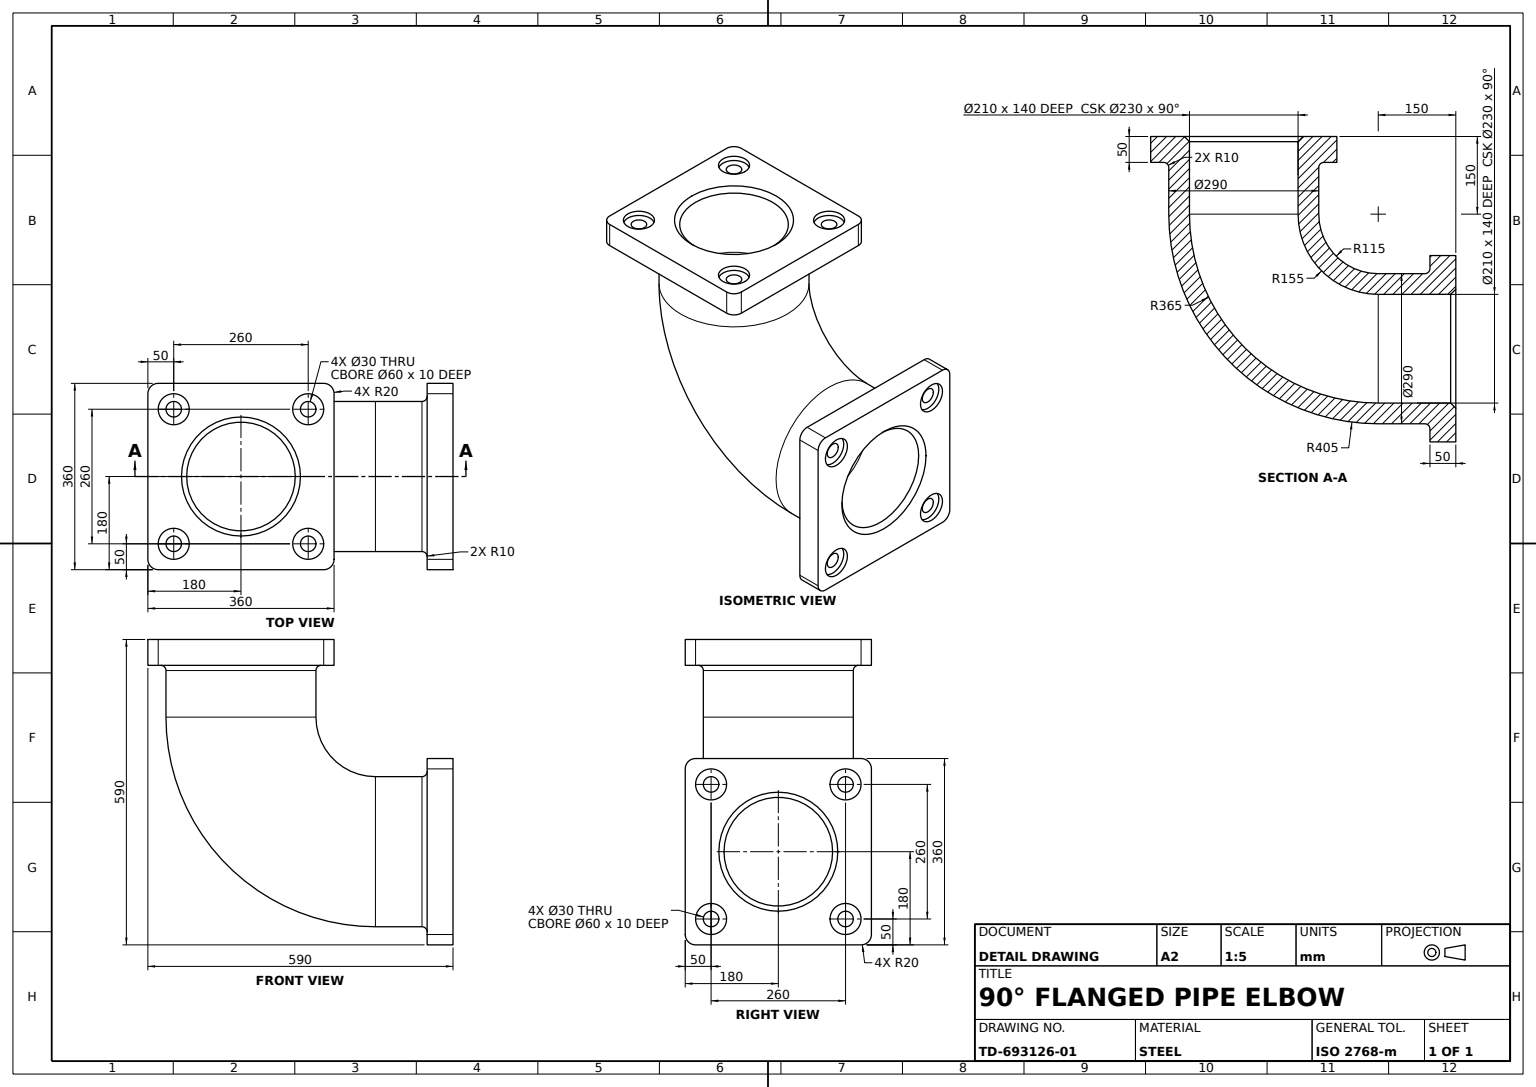
solid
v1 (0,260,215)
v2 (0,260,505)
e1 v1 v2 CIRCLE(AX(P(0,260,360),D(0,1,0),D(0,0,1)),145)
v3 (0,145,100)
e2 v3 v1 CIRCLE(AX(P(0,260,100),D(-1,0,0),D(0,0,1)),115)
v4 (0,-145,100)
e3 v3 v4 CIRCLE(AX(P(0,0,100),D(0,0,1),D(0,-1,0)),145)
e4 v4 v2 CIRCLE(AX(P(0,260,100),D(-1,0,0),D(0,0,1)),405)
face TORUS(AX(P(0,260,100),D(-1,0,0),D(0,0,1)),260,145) [-e1 -e2 e3 e4]
v5 (-100,130,-40)
v6 (-160,130,-40)
e5 v5 v6 CIRCLE(AX(P(-130,130,-40),D(0,0,-1),D(-1,0,0)),30)
v7 (-100,130,-50)
e6 v5 v7 LINE
v8 (-160,130,-50)
e7 v7 v8 CIRCLE(AX(P(-130,130,-50),D(0,0,-1),D(-1,0,0)),30)
e8 v6 v8 LINE
face CYL(AX(P(-130,130,-40),D(0,0,-1),D(-1,0,0)),30) rev [-e5 e6 e7 -e8]
e9 v6 v5 CIRCLE(AX(P(-130,130,-40),D(0,0,-1),D(-1,0,0)),30)
e10 v8 v7 CIRCLE(AX(P(-130,130,-50),D(0,0,-1),D(-1,0,0)),30)
face CYL(AX(P(-130,130,-40),D(0,0,-1),D(-1,0,0)),30) rev [-e9 e8 e10 -e6]
v9 (-130,400,200)
v10 (-130,410,200)
e11 v9 v10 LINE
v11 (-130,400,260)
e12 v11 v9 CIRCLE(AX(P(-130,400,230),D(0,1,0),D(0,0,1)),30)
v12 (-130,410,260)
e13 v11 v12 LINE
e14 v12 v10 CIRCLE(AX(P(-130,410,230),D(0,1,0),D(0,0,1)),30)
face CYL(AX(P(-130,400,230),D(0,1,0),D(0,0,1)),30) rev [-e11 -e12 e13 e14]
v13 (-130,400,520)
v14 (-130,400,460)
e15 v13 v14 CIRCLE(AX(P(-130,400,490),D(0,1,0),D(0,0,1)),30)
v15 (-130,410,520)
e16 v13 v15 LINE
v16 (-130,410,460)
e17 v15 v16 CIRCLE(AX(P(-130,410,490),D(0,1,0),D(0,0,1)),30)
e18 v14 v16 LINE
face CYL(AX(P(-130,400,490),D(0,1,0),D(0,0,1)),30) rev [-e15 e16 e17 -e18]
e19 v14 v13 CIRCLE(AX(P(-130,400,490),D(0,1,0),D(0,0,1)),30)
v17 (-130,400,505)
v18 (-130,400,475)
e20 v17 v18 CIRCLE(AX(P(-130,400,490),D(0,1,0),D(0,0,1)),15)
e21 v18 v17 CIRCLE(AX(P(-130,400,490),D(0,1,0),D(0,0,1)),15)
face PLANE(AX(P(-130,400,490),D(0,1,0),D(0,0,1))) [e19 e15] [-e20 -e21]
v19 (-180,-160,-50)
v20 (-180,-160,0)
e22 v19 v20 LINE
v21 (-180,160,0)
e23 v21 v20 LINE
v22 (-180,160,-50)
e24 v21 v22 LINE
e25 v22 v19 LINE
face PLANE(AX(P(-180,180,-50),D(-1,0,0),D(0,-1,0))) [e22 -e23 e24 e25]
v23 (-130,360,475)
e26 v18 v23 LINE
v24 (-130,360,505)
e27 v24 v23 CIRCLE(AX(P(-130,360,490),D(0,1,0),D(0,0,1)),15)
e28 v17 v24 LINE
face CYL(AX(P(-130,410,490),D(0,-1,0),D(0,0,-1)),15) rev [e20 e26 -e27 -e28]
v25 (130,400,200)
v26 (130,410,200)
e29 v25 v26 LINE
v27 (130,400,260)
e30 v27 v25 CIRCLE(AX(P(130,400,230),D(0,1,0),D(0,0,1)),30)
v28 (130,410,260)
e31 v27 v28 LINE
e32 v28 v26 CIRCLE(AX(P(130,410,230),D(0,1,0),D(0,0,1)),30)
face CYL(AX(P(130,400,230),D(0,1,0),D(0,0,1)),30) rev [-e29 -e30 e31 e32]
v29 (0,350,215)
e33 v1 v29 LINE
v30 (0,350,505)
e34 v2 v30 LINE
e35 v30 v29 CIRCLE(AX(P(0,350,360),D(0,-1,0),D(0,0,1)),145)
face CYL(AX(P(0,260,360),D(0,1,0),D(0,0,1)),145) [-e33 e1 e34 e35]
v31 (-115,-130,-40)
v32 (-145,-130,-40)
e36 v31 v32 CIRCLE(AX(P(-130,-130,-40),D(0,0,1),D(-1,0,0)),15)
v33 (-115,-130,0)
e37 v31 v33 LINE
v34 (-145,-130,0)
e38 v33 v34 CIRCLE(AX(P(-130,-130,0),D(0,0,1),D(1,0,0)),15)
e39 v32 v34 LINE
face CYL(AX(P(-130,-130,-50),D(0,0,1),D(1,0,0)),15) rev [-e36 e37 e38 -e39]
v35 (115,0,-50)
v36 (-115,0,-50)
e40 v35 v36 CIRCLE(AX(P(0,0,-50),D(0,0,1),D(1,0,0)),115)
v37 (105,0,-40)
e41 v37 v35 LINE
v38 (-105,0,-40)
e42 v38 v37 CIRCLE(AX(P(0,0,-40),D(0,0,-1),D(1,0,0)),105)
e43 v38 v36 LINE
face CONE(AX(P(0,0,-50),D(0,0,-1),D(-1,0,0)),115,0.785398163) rev [-e40 -e41 -e42 e43]
v39 (160,130,-40)
v40 (100,130,-40)
e44 v39 v40 CIRCLE(AX(P(130,130,-40),D(0,0,-1),D(-1,0,0)),30)
v41 (160,130,-50)
e45 v39 v41 LINE
v42 (100,130,-50)
e46 v41 v42 CIRCLE(AX(P(130,130,-50),D(0,0,-1),D(-1,0,0)),30)
e47 v40 v42 LINE
face CYL(AX(P(130,130,-40),D(0,0,-1),D(-1,0,0)),30) rev [-e44 e45 e46 -e47]
v43 (180,410,520)
v44 (180,410,200)
e48 v43 v44 LINE
v45 (160,410,180)
e49 v44 v45 CIRCLE(AX(P(160,410,200),D(0,1,0),D(0,0,1)),20)
v46 (-160,410,180)
e50 v45 v46 LINE
v47 (-180,410,200)
e51 v46 v47 CIRCLE(AX(P(-160,410,200),D(0,1,0),D(0,0,1)),20)
v48 (-180,410,520)
e52 v47 v48 LINE
v49 (-160,410,540)
e53 v48 v49 CIRCLE(AX(P(-160,410,520),D(0,1,0),D(0,0,1)),20)
v50 (160,410,540)
e54 v49 v50 LINE
e55 v50 v43 CIRCLE(AX(P(160,410,520),D(0,1,0),D(0,0,1)),20)
e56 v10 v12 CIRCLE(AX(P(-130,410,230),D(0,1,0),D(0,0,1)),30)
v51 (130,410,520)
v52 (130,410,460)
e57 v51 v52 CIRCLE(AX(P(130,410,490),D(0,1,0),D(0,0,1)),30)
e58 v52 v51 CIRCLE(AX(P(130,410,490),D(0,1,0),D(0,0,1)),30)
e59 v26 v28 CIRCLE(AX(P(130,410,230),D(0,1,0),D(0,0,1)),30)
v53 (0,410,245)
v54 (0,410,475)
e60 v53 v54 CIRCLE(AX(P(0,410,360),D(0,-1,0),D(0,0,1)),115)
e61 v54 v53 CIRCLE(AX(P(0,410,360),D(0,-1,0),D(0,0,1)),115)
e62 v16 v15 CIRCLE(AX(P(-130,410,490),D(0,1,0),D(0,0,1)),30)
face PLANE(AX(P(0,410,0),D(0,1,0),D(0,0,1))) [e48 e49 e50 e51 e52 e53 e54 e55] [-e56 -e14] [-e57 -e58] [-e59 -e32] [e60 e61] [-e17 -e62]
v55 (105,0,100)
e63 v37 v55 LINE
v56 (0,105,100)
e64 v56 v55 CIRCLE(AX(P(0,0,100),D(0,0,-1),D(0,-1,0)),105)
v57 (-105,0,100)
e65 v57 v56 CIRCLE(AX(P(0,0,100),D(0,0,-1),D(0,-1,0)),105)
e66 v38 v57 LINE
face CYL(AX(P(0,0,-50),D(0,0,1),D(1,0,0)),105) rev [e42 e63 -e64 -e65 -e66]
v58 (0,-105,100)
v59 (0,260,465)
e67 v58 v59 CIRCLE(AX(P(0,260,100),D(-1,0,0),D(0,0,1)),365)
v60 (0,260,255)
e68 v60 v59 CIRCLE(AX(P(0,260,360),D(0,-1,0),D(0,0,1)),105)
e69 v56 v60 CIRCLE(AX(P(0,260,100),D(-1,0,0),D(0,0,1)),155)
e70 v55 v58 CIRCLE(AX(P(0,0,100),D(0,0,-1),D(0,-1,0)),105)
face TORUS(AX(P(0,260,100),D(-1,0,0),D(0,0,1)),260,105) rev [e67 -e68 -e69 e64 e70]
e71 v37 v38 CIRCLE(AX(P(0,0,-40),D(0,0,-1),D(1,0,0)),105)
e72 v36 v35 CIRCLE(AX(P(0,0,-50),D(0,0,1),D(1,0,0)),115)
face CONE(AX(P(0,0,-50),D(0,0,-1),D(-1,0,0)),115,0.785398163) rev [-e71 e41 -e72 -e43]
v61 (0,360,205)
v62 (0,360,515)
e73 v61 v62 CIRCLE(AX(P(0,360,360),D(0,1,0),D(0,0,1)),155)
e74 v61 v29 CIRCLE(AX(P(0,350,205),D(1,0,0),D(0,0,-1)),10)
e75 v62 v30 CIRCLE(AX(P(0,350,515),D(-1,0,0),D(0,0,1)),10)
face TORUS(AX(P(0,350,360),D(0,1,0),D(0,0,1)),155,10) rev [-e73 e74 -e35 -e75]
v63 (160,180,0)
v64 (160,180,-50)
e76 v63 v64 LINE
v65 (-160,180,-50)
e77 v64 v65 LINE
v66 (-160,180,0)
e78 v65 v66 LINE
e79 v63 v66 LINE
face PLANE(AX(P(-180,180,-50),D(0,1,0),D(0,0,1))) [e76 e77 e78 -e79]
v67 (-160,-180,0)
v68 (-160,-180,-50)
e80 v67 v68 LINE
v69 (160,-180,-50)
e81 v68 v69 LINE
v70 (160,-180,0)
e82 v69 v70 LINE
e83 v67 v70 LINE
face PLANE(AX(P(-180,-180,-50),D(0,-1,0),D(0,0,-1))) [e80 e81 e82 -e83]
e84 v59 v60 CIRCLE(AX(P(0,260,360),D(0,-1,0),D(0,0,1)),105)
e85 v58 v57 CIRCLE(AX(P(0,0,100),D(0,0,-1),D(0,-1,0)),105)
face TORUS(AX(P(0,260,100),D(-1,0,0),D(0,0,1)),260,105) rev [e65 e69 -e84 -e67 e85]
v71 (0,-145,10)
v72 (145,0,10)
e86 v71 v72 CIRCLE(AX(P(0,0,10),D(0,0,1),D(1,0,0)),145)
v73 (0,145,10)
e87 v72 v73 CIRCLE(AX(P(0,0,10),D(0,0,1),D(1,0,0)),145)
e88 v73 v3 LINE
e89 v4 v3 CIRCLE(AX(P(0,0,100),D(0,0,1),D(0,-1,0)),145)
e90 v71 v4 LINE
face CYL(AX(P(0,0,0),D(0,0,1),D(0,-1,0)),145) [e86 e87 e88 -e89 -e90]
v74 (-160,360,540)
v75 (-180,360,520)
e91 v74 v75 CIRCLE(AX(P(-160,360,520),D(0,-1,0),D(0,0,1)),20)
e92 v49 v74 LINE
e93 v75 v48 LINE
face CYL(AX(P(-160,410,520),D(0,-1,0),D(0,0,-1)),20) [-e91 -e92 -e53 -e93]
v76 (145,130,0)
v77 (115,130,0)
e94 v76 v77 CIRCLE(AX(P(130,130,0),D(0,0,1),D(1,0,0)),15)
v78 (115,130,-40)
e95 v78 v77 LINE
v79 (145,130,-40)
e96 v79 v78 CIRCLE(AX(P(130,130,-40),D(0,0,1),D(-1,0,0)),15)
e97 v79 v76 LINE
face CYL(AX(P(130,130,-50),D(0,0,1),D(1,0,0)),15) rev [e94 -e95 -e96 e97]
e98 v23 v24 CIRCLE(AX(P(-130,360,490),D(0,1,0),D(0,0,1)),15)
face CYL(AX(P(-130,410,490),D(0,-1,0),D(0,0,-1)),15) rev [e21 e28 -e98 -e26]
v80 (100,-130,-40)
v81 (160,-130,-40)
e99 v80 v81 CIRCLE(AX(P(130,-130,-40),D(0,0,-1),D(-1,0,0)),30)
e100 v81 v80 CIRCLE(AX(P(130,-130,-40),D(0,0,-1),D(-1,0,0)),30)
v82 (115,-130,-40)
v83 (145,-130,-40)
e101 v82 v83 CIRCLE(AX(P(130,-130,-40),D(0,0,1),D(-1,0,0)),15)
e102 v83 v82 CIRCLE(AX(P(130,-130,-40),D(0,0,1),D(-1,0,0)),15)
face PLANE(AX(P(130,-130,-40),D(0,0,-1),D(-1,0,0))) [e99 e100] [e101 e102]
v84 (160,360,540)
e103 v84 v50 LINE
v85 (180,360,520)
e104 v85 v84 CIRCLE(AX(P(160,360,520),D(0,-1,0),D(0,0,1)),20)
e105 v43 v85 LINE
face CYL(AX(P(160,410,520),D(0,-1,0),D(0,0,-1)),20) [-e103 -e104 -e105 -e55]
e106 v42 v41 CIRCLE(AX(P(130,130,-50),D(0,0,-1),D(-1,0,0)),30)
e107 v68 v19 CIRCLE(AX(P(-160,-160,-50),D(0,0,-1),D(1,0,0)),20)
e108 v22 v65 CIRCLE(AX(P(-160,160,-50),D(0,0,-1),D(1,0,0)),20)
v86 (180,160,-50)
e109 v64 v86 CIRCLE(AX(P(160,160,-50),D(0,0,-1),D(1,0,0)),20)
v87 (180,-160,-50)
e110 v87 v86 LINE
e111 v87 v69 CIRCLE(AX(P(160,-160,-50),D(0,0,-1),D(1,0,0)),20)
v88 (160,-130,-50)
v89 (100,-130,-50)
e112 v88 v89 CIRCLE(AX(P(130,-130,-50),D(0,0,-1),D(-1,0,0)),30)
e113 v89 v88 CIRCLE(AX(P(130,-130,-50),D(0,0,-1),D(-1,0,0)),30)
v90 (-160,-130,-50)
v91 (-100,-130,-50)
e114 v90 v91 CIRCLE(AX(P(-130,-130,-50),D(0,0,-1),D(-1,0,0)),30)
e115 v91 v90 CIRCLE(AX(P(-130,-130,-50),D(0,0,-1),D(-1,0,0)),30)
face PLANE(AX(P(0,0,-50),D(0,0,1),D(1,0,0))) rev [-e106 -e46] [e40 e72] [e107 -e25 e108 -e77 e109 -e110 e111 -e81] [-e7 -e10] [-e112 -e113] [-e114 -e115]
v92 (0,400,255)
e116 v92 v53 LINE
v93 (0,400,465)
e117 v93 v54 LINE
e118 v92 v93 CIRCLE(AX(P(0,400,360),D(0,1,0),D(0,0,1)),105)
face CONE(AX(P(0,400,360),D(0,1,0),D(0,0,1)),105,0.785398163) rev [e116 -e61 -e117 -e118]
v94 (-160,-130,-40)
v95 (-100,-130,-40)
e119 v94 v95 CIRCLE(AX(P(-130,-130,-40),D(0,0,-1),D(-1,0,0)),30)
e120 v94 v90 LINE
e121 v95 v91 LINE
face CYL(AX(P(-130,-130,-40),D(0,0,-1),D(-1,0,0)),30) rev [-e119 e120 e114 -e121]
e122 v40 v39 CIRCLE(AX(P(130,130,-40),D(0,0,-1),D(-1,0,0)),30)
face CYL(AX(P(130,130,-40),D(0,0,-1),D(-1,0,0)),30) rev [-e45 -e122 e47 e106]
e123 v32 v31 CIRCLE(AX(P(-130,-130,-40),D(0,0,1),D(-1,0,0)),15)
e124 v95 v94 CIRCLE(AX(P(-130,-130,-40),D(0,0,-1),D(-1,0,0)),30)
face PLANE(AX(P(-130,-130,-40),D(0,0,-1),D(-1,0,0))) [e36 e123] [e119 e124]
e125 v29 v30 CIRCLE(AX(P(0,350,360),D(0,-1,0),D(0,0,1)),145)
e126 v2 v1 CIRCLE(AX(P(0,260,360),D(0,1,0),D(0,0,1)),145)
face CYL(AX(P(0,260,360),D(0,1,0),D(0,0,1)),145) [e125 -e34 e126 e33]
e127 v20 v67 CIRCLE(AX(P(-160,-160,0),D(0,0,1),D(1,0,0)),20)
face CYL(AX(P(-160,-160,-50),D(0,0,1),D(1,0,0)),20) [-e107 -e80 -e127 -e22]
v96 (180,160,0)
e128 v86 v96 LINE
v97 (180,-160,0)
e129 v97 v96 LINE
e130 v97 v87 LINE
face PLANE(AX(P(180,180,-50),D(1,0,0),D(0,1,0))) [e110 e128 -e129 e130]
face TORUS(AX(P(0,260,100),D(-1,0,0),D(0,0,1)),260,145) [-e126 -e4 e89 e2]
e131 v81 v88 LINE
e132 v80 v89 LINE
face CYL(AX(P(130,-130,-40),D(0,0,-1),D(-1,0,0)),30) rev [-e100 e131 e112 -e132]
v98 (130,400,215)
v99 (130,360,215)
e133 v98 v99 LINE
v100 (130,360,245)
e134 v100 v99 CIRCLE(AX(P(130,360,230),D(0,1,0),D(0,0,1)),15)
v101 (130,400,245)
e135 v101 v100 LINE
e136 v101 v98 CIRCLE(AX(P(130,400,230),D(0,1,0),D(0,0,1)),15)
face CYL(AX(P(130,410,230),D(0,-1,0),D(0,0,-1)),15) rev [e133 -e134 -e135 e136]
face CYL(AX(P(-130,-130,-40),D(0,0,-1),D(-1,0,0)),30) rev [e121 e115 -e120 -e124]
face CYL(AX(P(0,0,-50),D(0,0,1),D(1,0,0)),105) rev [-e85 -e70 -e63 e71 e66]
e137 v66 v21 CIRCLE(AX(P(-160,160,0),D(0,0,1),D(1,0,0)),20)
face CYL(AX(P(-160,160,-50),D(0,0,1),D(1,0,0)),20) [-e78 -e108 -e24 -e137]
e138 v59 v93 LINE
e139 v60 v92 LINE
face CYL(AX(P(0,260,360),D(0,1,0),D(0,0,1)),105) rev [e118 -e138 e84 e139]
v102 (160,360,180)
e140 v45 v102 LINE
v103 (-160,360,180)
e141 v102 v103 LINE
e142 v103 v46 LINE
face PLANE(AX(P(-180,410,180),D(0,0,1),D(1,0,0))) rev [e140 e141 e142 -e50]
e143 v34 v33 CIRCLE(AX(P(-130,-130,0),D(0,0,1),D(1,0,0)),15)
face CYL(AX(P(-130,-130,-50),D(0,0,1),D(1,0,0)),15) rev [e143 -e37 -e123 e39]
v104 (130,400,475)
v105 (130,360,475)
e144 v104 v105 LINE
v106 (130,360,505)
e145 v106 v105 CIRCLE(AX(P(130,360,490),D(0,1,0),D(0,0,1)),15)
v107 (130,400,505)
e146 v107 v106 LINE
e147 v107 v104 CIRCLE(AX(P(130,400,490),D(0,1,0),D(0,0,1)),15)
face CYL(AX(P(130,410,490),D(0,-1,0),D(0,0,-1)),15) rev [e144 -e145 -e146 e147]
v108 (-130,400,215)
v109 (-130,400,245)
e148 v108 v109 CIRCLE(AX(P(-130,400,230),D(0,1,0),D(0,0,1)),15)
v110 (-130,360,245)
e149 v109 v110 LINE
v111 (-130,360,215)
e150 v111 v110 CIRCLE(AX(P(-130,360,230),D(0,1,0),D(0,0,1)),15)
e151 v108 v111 LINE
face CYL(AX(P(-130,410,230),D(0,-1,0),D(0,0,-1)),15) rev [e148 e149 -e150 -e151]
e152 v62 v61 CIRCLE(AX(P(0,360,360),D(0,1,0),D(0,0,1)),155)
face TORUS(AX(P(0,350,360),D(0,1,0),D(0,0,1)),155,10) rev [-e74 -e152 e75 -e125]
e153 v9 v11 CIRCLE(AX(P(-130,400,230),D(0,1,0),D(0,0,1)),30)
e154 v109 v108 CIRCLE(AX(P(-130,400,230),D(0,1,0),D(0,0,1)),15)
face PLANE(AX(P(-130,400,230),D(0,1,0),D(0,0,1))) [e12 e153] [-e148 -e154]
v112 (180,360,200)
e155 v112 v44 LINE
e156 v85 v112 LINE
face PLANE(AX(P(180,410,180),D(-1,0,0),D(0,0,1))) rev [e155 -e48 e105 e156]
e157 v99 v100 CIRCLE(AX(P(130,360,230),D(0,1,0),D(0,0,1)),15)
e158 v98 v101 CIRCLE(AX(P(130,400,230),D(0,1,0),D(0,0,1)),15)
face CYL(AX(P(130,410,230),D(0,-1,0),D(0,0,-1)),15) rev [e135 -e157 -e133 e158]
v113 (-115,130,-40)
v114 (-145,130,-40)
e159 v113 v114 CIRCLE(AX(P(-130,130,-40),D(0,0,1),D(-1,0,0)),15)
v115 (-115,130,0)
e160 v113 v115 LINE
v116 (-145,130,0)
e161 v115 v116 CIRCLE(AX(P(-130,130,0),D(0,0,1),D(1,0,0)),15)
e162 v114 v116 LINE
face CYL(AX(P(-130,130,-50),D(0,0,1),D(1,0,0)),15) rev [-e159 e160 e161 -e162]
v117 (-180,360,200)
e163 v117 v103 CIRCLE(AX(P(-160,360,200),D(0,-1,0),D(0,0,1)),20)
e164 v47 v117 LINE
face CYL(AX(P(-160,410,200),D(0,-1,0),D(0,0,-1)),20) [-e163 -e164 -e51 -e142]
e165 v70 v97 CIRCLE(AX(P(160,-160,0),D(0,0,1),D(1,0,0)),20)
face CYL(AX(P(160,-160,-50),D(0,0,1),D(1,0,0)),20) [-e82 -e111 -e130 -e165]
face CYL(AX(P(130,-130,-40),D(0,0,-1),D(-1,0,0)),30) rev [e113 -e131 -e99 e132]
e166 v116 v115 CIRCLE(AX(P(-130,130,0),D(0,0,1),D(1,0,0)),15)
e167 v114 v113 CIRCLE(AX(P(-130,130,-40),D(0,0,1),D(-1,0,0)),15)
face CYL(AX(P(-130,130,-50),D(0,0,1),D(1,0,0)),15) rev [e166 -e160 -e167 e162]
e168 v105 v106 CIRCLE(AX(P(130,360,490),D(0,1,0),D(0,0,1)),15)
e169 v117 v75 LINE
e170 v102 v112 CIRCLE(AX(P(160,360,200),D(0,-1,0),D(0,0,1)),20)
e171 v74 v84 LINE
e172 v110 v111 CIRCLE(AX(P(-130,360,230),D(0,1,0),D(0,0,1)),15)
face PLANE(AX(P(0,360,0),D(0,1,0),D(0,0,1))) rev [e152 e73] [e168 e145] [e91 -e169 e163 -e141 e170 -e156 e104 -e171] [e172 e150] [e134 e157] [e98 e27]
face CYL(AX(P(-130,400,230),D(0,1,0),D(0,0,1)),30) rev [-e153 e11 e56 -e13]
face PLANE(AX(P(-180,410,540),D(0,0,-1),D(-1,0,0))) rev [e92 e171 e103 -e54]
e173 v96 v63 CIRCLE(AX(P(160,160,0),D(0,0,1),D(1,0,0)),20)
v118 (155,0,0)
v119 (-155,0,0)
e174 v118 v119 CIRCLE(AX(P(0,0,0),D(0,0,-1),D(1,0,0)),155)
e175 v119 v118 CIRCLE(AX(P(0,0,0),D(0,0,-1),D(1,0,0)),155)
e176 v77 v76 CIRCLE(AX(P(130,130,0),D(0,0,1),D(1,0,0)),15)
v120 (115,-130,0)
v121 (145,-130,0)
e177 v120 v121 CIRCLE(AX(P(130,-130,0),D(0,0,1),D(1,0,0)),15)
e178 v121 v120 CIRCLE(AX(P(130,-130,0),D(0,0,1),D(1,0,0)),15)
face PLANE(AX(P(0,0,0),D(0,0,1),D(1,0,0))) [-e143 -e38] [-e161 -e166] [e165 e129 e173 e79 e137 e23 e127 e83] [e174 e175] [-e176 -e94] [-e177 -e178]
e179 v25 v27 CIRCLE(AX(P(130,400,230),D(0,1,0),D(0,0,1)),30)
face CYL(AX(P(130,400,230),D(0,1,0),D(0,0,1)),30) rev [-e31 -e179 e29 e59]
face CYL(AX(P(160,160,-50),D(0,0,1),D(1,0,0)),20) [-e173 -e128 -e109 -e76]
face CYL(AX(P(160,410,200),D(0,-1,0),D(0,0,-1)),20) [-e155 -e170 -e140 -e49]
v122 (-145,0,10)
e180 v73 v122 CIRCLE(AX(P(0,0,10),D(0,0,1),D(1,0,0)),145)
e181 v122 v71 CIRCLE(AX(P(0,0,10),D(0,0,1),D(1,0,0)),145)
face CYL(AX(P(0,0,0),D(0,0,1),D(0,-1,0)),145) [-e88 e180 e181 e90 -e3]
e182 v93 v92 CIRCLE(AX(P(0,400,360),D(0,1,0),D(0,0,1)),105)
face CONE(AX(P(0,400,360),D(0,1,0),D(0,0,1)),105,0.785398163) rev [-e116 -e182 e117 -e60]
e183 v72 v118 CIRCLE(AX(P(155,0,10),D(0,-1,0),D(0,0,-1)),10)
e184 v122 v119 CIRCLE(AX(P(-155,0,10),D(0,1,0),D(-1,0,0)),10)
face TORUS(AX(P(0,0,10),D(0,0,1),D(1,0,0)),155,10) rev [-e180 -e87 e183 -e175 -e184]
face PLANE(AX(P(-130,130,-40),D(0,0,-1),D(-1,0,0))) [e9 e5] [e159 e167]
v123 (130,400,520)
v124 (130,400,460)
e185 v123 v124 CIRCLE(AX(P(130,400,490),D(0,1,0),D(0,0,1)),30)
e186 v124 v123 CIRCLE(AX(P(130,400,490),D(0,1,0),D(0,0,1)),30)
e187 v104 v107 CIRCLE(AX(P(130,400,490),D(0,1,0),D(0,0,1)),15)
face PLANE(AX(P(130,400,490),D(0,1,0),D(0,0,1))) [e185 e186] [-e147 -e187]
face CYL(AX(P(-130,410,230),D(0,-1,0),D(0,0,-1)),15) rev [-e172 -e149 e154 e151]
face PLANE(AX(P(130,400,230),D(0,1,0),D(0,0,1))) [e30 e179] [-e158 -e136]
e188 v78 v79 CIRCLE(AX(P(130,130,-40),D(0,0,1),D(-1,0,0)),15)
face PLANE(AX(P(130,130,-40),D(0,0,-1),D(-1,0,0))) [e96 e188] [e44 e122]
e189 v124 v52 LINE
e190 v123 v51 LINE
face CYL(AX(P(130,400,490),D(0,1,0),D(0,0,1)),30) rev [e189 e58 -e190 -e186]
face CYL(AX(P(-130,400,490),D(0,1,0),D(0,0,1)),30) rev [e18 e62 -e16 -e19]
face CYL(AX(P(130,400,490),D(0,1,0),D(0,0,1)),30) rev [-e189 -e185 e190 e57]
e191 v83 v121 LINE
e192 v82 v120 LINE
face CYL(AX(P(130,-130,-50),D(0,0,1),D(1,0,0)),15) rev [e191 e178 -e192 -e102]
face CYL(AX(P(130,410,490),D(0,-1,0),D(0,0,-1)),15) rev [e187 e146 -e168 -e144]
face CYL(AX(P(0,260,360),D(0,1,0),D(0,0,1)),105) rev [e68 e138 e182 -e139]
face CYL(AX(P(130,-130,-50),D(0,0,1),D(1,0,0)),15) rev [e177 -e191 -e101 e192]
face PLANE(AX(P(-180,410,180),D(1,0,0),D(0,0,-1))) rev [e93 -e52 e164 e169]
face CYL(AX(P(130,130,-50),D(0,0,1),D(1,0,0)),15) rev [e95 e176 -e97 -e188]
face TORUS(AX(P(0,0,10),D(0,0,1),D(1,0,0)),155,10) rev [e184 -e174 -e183 -e86 -e181]
